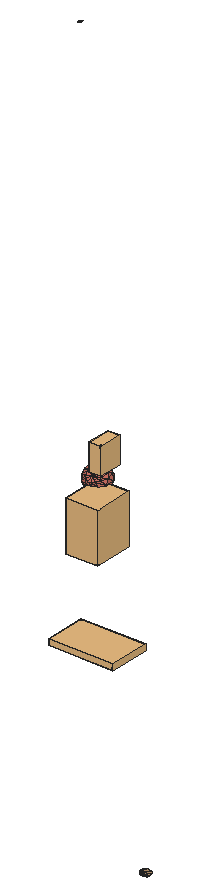
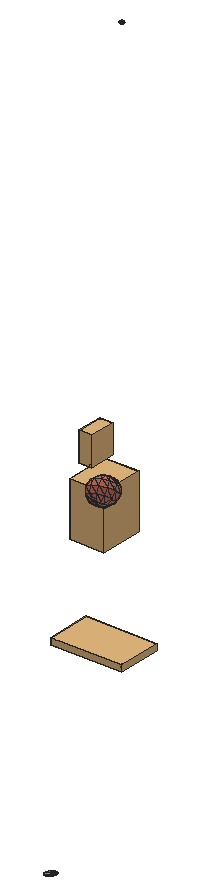
# SketchUp Ruby script. Lengths in inches.
U = 1.inch
M = Sketchup.active_model
def pt(a) = Geom::Point3d.new(a.map { |v| v * U })
def face(e, loops, mat)
  f = e.add_face(loops[0].map { |a| pt(a) })
  loops[1..].each { |l| e.add_face(l.map { |a| pt(a) }).erase! }
  f.material = f.back_material = mat if mat
  f
end
# faces: each face lists its corners as indices into pts; further lists are holes
def faces(e, pts, list, mat = nil) = list.each { |f| face(e, (f[0].is_a?(Array) ? f : [f]).map { |l| l.map { |i| pts[i] } }, mat) }
# xy, xz, yz: faces in a plane at the given z, y or x. An outline is a flat list of corners, or four numbers for a rectangle; further outlines are holes
def ring(l) = l.size == 4 ? [[l[0], l[1]], [l[2], l[1]], [l[2], l[3]], [l[0], l[3]]] : l.each_slice(2).to_a
def flat(e, list, mat, &to3) = list.each { |f| face(e, (f[0].is_a?(Array) ? f : [f]).map { |l| ring(l).map { |u, v| to3.(u, v) } }, mat) }
def xy(e, z, list, mat = nil) = flat(e, list, mat) { |x, y| [x, y, z] }
def xz(e, y, list, mat = nil) = flat(e, list, mat) { |x, z| [x, y, z] }
def yz(e, x, list, mat = nil) = flat(e, list, mat) { |y, z| [x, y, z] }
def lines(e, pts, list) = list.each { |a, b| e.add_line(pt(pts[a]), pt(pts[b])) }
# prism: a flat outline (further loops are holes) pulled along v
def prism(e, loops, v, mat = nil)
  f = face(e, loops, mat); d = Geom::Vector3d.new(v.map { |x| x * U })
  f.pushpull(f.normal.samedirection?(d) ? d.length : -d.length)
end
def box(e, o, s, mat = nil) = prism(e, [[o, [o[0] + s[0], o[1], o[2]], [o[0] + s[0], o[1] + s[1], o[2]], [o[0], o[1] + s[1], o[2]]]], [0, 0, s[2]], mat)
def at(x, y, z, deg = 0) = Geom::Transformation.translation(pt([x, y, z])) * Geom::Transformation.rotation(ORIGIN, Z_AXIS, deg.degrees)
def axes(o, x, y, z) = Geom::Transformation.new([*x, 0, *y, 0, *z, 0, *pt(o).to_a, 1])
def part(name) = M.definitions.add(name)
# library, detail: a bought-in or finely detailed component or shape, given as its bounding box
def library(name, o, s) = part(name).tap { |d| box(d.entities, o, s) }
def detail(e, o, s) = box(e.add_group.entities, o, s)
def put(e, d, t, mat = nil) = e.add_instance(d, t).tap { |i| i.material = mat if mat }
def group(e, t, mat = nil) = e.add_group.tap { |g| g.transformation = t; g.material = mat if mat }.entities
root = M.entities
M.materials.add("green").color = [174, 139, 102]
M.materials.add("vio").color = [206, 114, 100]
c1 = part("3DGeom~213_Defintion")
p = [[-61.03,-133.26,-481.34],[151.11,0,-487.05],[280.8,-170.5625,-375.28],[435.08,-14.45,-265.46],[280.8,-170.5625,-375.28],[-208.41,14.45,-465.11],
  [322.77,133.26,-362.26],[435.08,-14.45,-265.46],[-19.0625,170.56,-468.3125],[-256.82,-230.81,-346.65],[51.28,-280.97,-384.54],[280.8,-170.5625,-375.28],
  [51.28,-280.97,-384.54],[-341.91,-145.53,-337.28],[-256.82,-230.81,-346.65],[-341.91,-145.53,-337.28],[-351.36,122.58,-340.21],[-184.13,295.42,-324.09],
  [175.39,280.97,-346.03],[-424.44,-83.1,-265.17],[-341.91,-145.53,-337.28],[-424.44,-83.1,-265.17],[-191.98,-316.09,-290.76],[51.28,-280.97,-384.54],
  [98.43,-389.1,-200.66],[335.24,-295.42,-162.95],[-256.82,-230.81,-346.65],[51.28,-280.97,-384.54],[-191.98,-316.09,-290.76],[280.8,-170.5625,-375.28],
  [280.8,-170.5625,-375.28],[482.23,-122.58,-81.58],[335.24,-295.42,-162.95],[280.8,-170.5625,-375.28],[435.08,-14.45,-265.46],[322.77,133.26,-362.26],
  [472.78,145.53,-84.51],[175.39,280.97,-346.03],[407.9375,230.81,-140.4],[322.77,133.26,-362.26],[322.77,133.26,-362.26],[-256.82,-230.81,-346.65],
  [-191.98,-316.09,-290.76],[-383.8,-266.51,-119.08],[-341.91,-145.53,-337.28],[-383.8,-266.51,-119.08],[175.39,280.97,-346.03],[322.85,316.09,-131.03],
  [32.44,389.1,-221.13],[32.44,389.1,-221.13],[322.85,316.09,-131.03],[175.39,280.97,-346.03],[-482.31,-60.25,-149.64],[-351.36,122.58,-340.21],
  [-424.44,-83.1,-265.17],[-451.58,162.16,-140.11],[-351.36,122.58,-340.21],[-184.13,295.42,-324.09],[-351.36,122.58,-340.21],[-383.8,-266.51,-119.08],
  [-299.86,341.12,-93.03],[-184.13,295.42,-324.09],[-299.86,341.12,-93.03],[32.44,389.1,-221.13],[-184.13,295.42,-324.09],[-164.76,-378.52,-184.6],
  [-383.8,-266.51,-119.08],[500,83.1,21.65],[-383.8,-266.51,-119.08],[32.44,389.1,-221.13],[240.32,378.52,-58.92],[322.85,316.09,-131.03],
  [-299.86,341.12,-93.03],[-67.78,428.68,-21.03],[32.44,389.1,-221.13],[32.44,389.1,-221.13],[67.78,-428.68,21.03],[299.86,-341.12,93.03],
  [-182.45,-401.37,-56.61],[335.24,-295.42,-162.95],[451.58,-162.16,140.11],[299.86,-341.12,93.03],[335.24,-295.42,-162.95],[-500,-83.1,-21.65],
  [-383.8,-266.51,-119.08],[383.8,266.51,119.08],[-482.23,122.58,81.58],[240.32,378.52,-58.92],[-240.32,-378.52,58.92],[-240.32,-378.52,58.92],
  [-322.85,-316.09,131.03],[-383.8,-266.51,-119.08],[-407.9375,-230.81,140.4],[-383.8,-266.51,-119.08],[-472.78,-145.53,84.51],[-383.8,-266.51,-119.08],
  [-383.8,-266.51,-119.08],[-335.24,295.42,162.95],[-335.24,295.42,162.95],[-299.86,341.12,-93.03],[482.31,60.25,149.64],[182.45,401.37,56.61],
  [383.8,266.51,119.08],[-32.44,-389.1,221.14],[-240.32,-378.52,58.92],[-335.24,295.42,162.95],[-98.43,389.1,200.66],[184.13,-295.42,324.09],
  [184.13,-295.42,324.09],[164.76,378.52,184.6],[383.8,266.51,119.08],[-240.32,-378.52,58.92],[-175.39,-280.97,346.03],[-240.32,-378.52,58.92],
  [-175.39,-280.97,346.03],[-322.85,-316.09,131.03],[-435.08,14.45,265.46],[299.86,-341.12,93.03],[351.36,-122.58,340.21],[184.13,-295.42,324.09],
  [299.86,-341.12,93.03],[351.36,-122.58,340.21],[424.44,83.1,265.17],[341.91,145.53,337.28],[424.44,83.1,265.17],[256.82,230.81,346.65],
  [341.91,145.53,337.28],[191.98,316.09,290.76],[256.82,230.81,346.65],[191.98,316.09,290.76],[383.8,266.51,119.08],[-322.77,-133.26,362.26],
  [-175.39,-280.97,346.03],[424.44,83.1,265.17],[351.36,-122.58,340.21],[424.44,83.1,265.17],[-280.8,170.5625,375.28],[-280.8,170.5625,375.28],
  [-335.24,295.42,162.95],[-51.28,280.97,384.54],[-280.8,170.5625,375.28],[-32.44,-389.1,221.14],[19.0625,-170.56,468.3125],[-175.39,-280.97,346.03],
  [-32.44,-389.1,221.14],[184.13,-295.42,324.09],[351.36,-122.58,340.21],[424.44,83.1,265.17],[341.91,145.53,337.28],[-322.77,-133.26,362.26],
  [-280.8,170.5625,375.28],[-435.08,14.45,265.46],[61.03,133.26,481.34],[191.98,316.09,290.76],[-51.28,280.97,384.54],[256.82,230.81,346.65],
  [191.98,316.09,290.76],[208.41,-14.45,465.11],[-175.39,-280.97,346.03],[-151.11,0,487.05],[-322.77,-133.26,362.26],[-175.39,-280.97,346.03],
  [-322.77,-133.26,362.26],[-280.8,170.5625,375.28],[-51.28,280.97,384.54],[-280.8,170.5625,375.28],[-51.28,280.97,384.54]]
faces(c1.entities,p,[[0,1,2],[1,3,4],[5,1,0],[1,6,7],[5,8,1],[8,6,1],[9,0,10],[0,11,12],
  [13,0,14],[15,5,0],[16,8,5],[16,17,8],[8,18,6],[17,18,8],[19,5,20],[21,16,5],
  [22,23,24],[23,25,24],[26,27,28],[23,29,25],[30,31,32],[33,34,31],[35,36,34],[37,38,39],
  [40,38,36],[41,42,43],[44,41,45],[46,47,38],[17,48,18],[49,50,51],[52,53,54],[52,55,56],
  [55,57,58],[54,44,59],[55,60,61],[62,63,64],[22,24,65],[22,65,66],[34,67,31],[34,36,67],
  [52,54,68],[69,70,71],[72,73,74],[73,70,75],[65,24,76],[24,77,76],[24,25,77],[65,76,78],
  [65,78,66],[79,80,81],[82,31,80],[83,52,84],[83,55,52],[36,38,85],[38,47,85],[83,86,55],
  [86,60,55],[47,87,85],[78,88,66],[89,90,91],[90,92,93],[94,83,95],[92,94,96],[86,97,60],
  [98,73,99],[67,36,85],[31,100,80],[31,67,100],[70,101,102],[73,101,70],[78,76,103],[78,103,104],
  [94,86,83],[105,106,73],[106,101,73],[76,107,103],[76,77,108],[100,67,85],[101,109,110],[106,109,101],
  [111,103,112],[113,114,115],[94,116,86],[116,97,86],[92,116,94],[117,118,119],[120,80,121],[122,100,85],
  [123,124,85],[125,126,85],[127,128,85],[109,129,130],[90,131,92],[90,132,131],[80,133,134],[80,100,135],
  [92,131,116],[116,136,97],[137,106,138],[139,109,106],[139,129,109],[140,139,106],[141,142,143],[144,145,142],
  [146,147,148],[149,150,151],[152,153,154],[152,155,156],[145,157,142],[145,146,157],[146,148,157],[157,148,155],
  [158,159,160],[161,142,159],[157,155,152],[162,159,163],[159,164,165],[159,152,166],[142,157,152],[142,152,159]],"vio")
c2 = library("3DGeom~82_Defintion",[-311.46,-44.07,-500],[622.92,88.14,1000])
c3 = part("3DGeom~83_Defintion")
p = [[-298.62,24.62,-492.72],[-284.8,11.4,-500],[-286.34,4.79,-498.51],[-298.62,24.62,-492.72],[-286.83,18.01,-499.32],[-284.8,11.4,-500],
  [-298.62,24.62,-492.72],[-291.89,22.84,-496.66],[-286.83,18.01,-499.32],[-298.62,24.62,-492.72],[-286.34,4.79,-498.51],[-291.04,-0.05,-495.25],
  [-298.62,24.62,-492.72],[-291.04,-0.05,-495.25],[-297.64,-1.82,-491.09],[-298.62,24.62,-492.72],[-297.64,-1.82,-491.09],[-304.37,-0.05,-487.15],
  [-298.62,24.62,-492.72],[-304.37,-0.05,-487.15],[-309.43,4.79,-484.49],[-298.62,24.62,-492.72],[-309.43,4.79,-484.49],[-311.46,11.4,-483.81],
  [-298.62,24.62,-492.72],[-311.46,11.4,-483.81],[-309.92,18.01,-485.3],[-298.62,24.62,-492.72],[-309.92,18.01,-485.3],[-305.22,22.84,-488.56],
  [307.6,-38.25,479.62],[301.85,-20.79,496.17],[294.12,-44.07,483.45],[307.6,-38.25,479.62],[294.12,-44.07,483.45],[301.3,-42.51,480.25],
  [311.46,-26.61,485.98],[301.85,-20.79,496.17],[307.6,-38.25,479.62],[311.46,-26.61,485.98],[307.6,-38.25,479.62],[311.32,-32.43,481.71],
  [294.12,-44.07,483.45],[301.85,-20.79,496.17],[284.51,-38.25,493.64],[294.12,-44.07,483.45],[284.51,-38.25,493.64],[287.97,-42.51,488.35],
  [301.85,-20.79,496.17],[311.46,-26.61,485.98],[307.99,-22.35,491.27],[284.51,-38.25,493.64],[301.85,-20.79,496.17],[288.37,-26.61,500],
  [284.51,-38.25,493.64],[284.65,-32.43,497.9],[301.85,-20.79,496.17],[294.66,-22.35,499.36]]
faces(c3.entities,p,[[0,1,2],[3,4,5],[6,7,8],[9,10,11],[12,13,14],[15,16,17],[18,19,20],[21,22,23],
  [24,25,26],[27,28,29],[30,31,32],[33,34,35],[36,37,38],[39,40,41],[42,43,44],[45,46,47],
  [48,49,50],[51,52,53],[54,53,55],[56,57,53]],"green")
c4 = library("3DGeom~150_Defintion",[-440.97,-500,-219.09],[881.94,1000,438.17])
c5 = part("3DGeom~151_Defintion")
p = [[-380.69,-485.53,-210.54],[-411.26,-467,-218.1875],[-394.16,-475.51,-219.09],[-380.69,-485.53,-210.54],[-434.74,-476.74,-157.14],[-411.26,-467,-218.1875],
  [-438.29,-462.61,-191.49],[-411.26,-467,-218.1875],[-438.29,-462.61,-191.49],[-427.41,-462.28,-208.09],[-377.14,-499.67,-176.1875],[-434.74,-476.74,-157.14],
  [-380.69,-485.53,-210.54],[-377.14,-499.67,-176.1875],[-380.69,-485.53,-210.54],[-374.46,-494.375,-194.84],[-434.74,-476.74,-157.14],[-440.97,-467.9,-172.84],
  [-438.29,-462.61,-191.49],[-404.17,-495.28,-149.49],[-377.14,-499.67,-176.1875],[-388.02,-500,-159.59],[-404.17,-495.28,-149.49],[-434.74,-476.74,-157.14],
  [-404.17,-495.28,-149.49],[-421.27,-486.76,-148.6],[402.51,492.03,208.37],[431.04,458.58,149.1],[419.28,470.25,140.94],[402.51,492.03,208.37],
  [419.28,470.25,140.94],[406.85,483.28,142.92],[402.51,492.03,208.37],[406.85,483.28,142.92],[397.08,494.17,154.49],[402.51,492.03,208.37],
  [438.98,451.39,165.19],[431.04,458.58,149.1],[402.51,492.03,208.37],[397.08,494.17,154.49],[392.58,500,172.55],[402.51,492.03,208.37],
  [440.97,450.61,184.92],[438.98,451.39,165.19],[402.51,492.03,208.37],[392.58,500,172.55],[394.57,499.22,192.28],[402.51,492.03,208.37],
  [436.48,456.44,202.98],[440.97,450.61,184.92],[402.51,492.03,208.37],[426.7,467.33,214.55],[402.51,492.03,208.37],[414.27,480.36,216.53],
  [426.7,467.33,214.55]]
faces(c5.entities,p,[[0,1,2],[3,4,5],[5,4,6],[7,8,9],[10,11,12],[13,14,15],[16,17,18],[19,20,21],
  [22,11,10],[23,24,25],[26,27,28],[29,30,31],[32,33,34],[35,36,37],[38,39,40],[41,42,43],
  [44,45,46],[47,48,49],[50,51,48],[52,53,54]],"green")
c6 = part("3DGeom~137_Defintion")
p = [[-12.7,499.9,-47.63],[-12.43,498.46,-37.01],[-9.46,500,-49.08],[-9.46,500,-49.08],[-12.43,498.46,-37.01],[-5.93,499.84,-48.71],
  [-9.46,500,-49.08],[-5.93,499.84,-48.71],[-7.64,499.95,-49.12],[-12.7,499.9,-47.63],[-9.46,500,-49.08],[-11.2,499.98,-48.56],
  [-5.93,499.84,-48.71],[-12.43,498.46,-37.01],[-3.15,499.49,-46.71],[-5.93,499.84,-48.71],[-3.15,499.49,-46.71],[-4.41,499.68,-47.89],
  [-13.6875,498.66,-38.1875],[-12.43,498.46,-37.01],[-12.7,499.9,-47.63],[-13.6875,498.66,-38.1875],[-12.7,499.9,-47.63],[-13.9,499.77,-46.38],
  [-3.15,499.49,-46.71],[-12.43,498.46,-37.01],[-1.7,499.01,-43.51],[-3.15,499.49,-46.71],[-1.7,499.01,-43.51],[-2.22,499.26,-45.24],
  [-15.16,499.38,-43.18],[-13.6875,498.66,-38.1875],[-13.9,499.77,-46.38],[-15.16,499.38,-43.18],[-13.9,499.77,-46.38],[-14.73,499.59,-44.87],
  [-1.7,499.01,-43.51],[-12.43,498.46,-37.01],[-2.1,498.55,-40.03],[-1.7,499.01,-43.51],[-2.1,498.55,-40.03],[-1.67,498.77,-41.72],
  [-15.13,499.14,-41.38],[-13.6875,498.66,-38.1875],[-15.16,499.38,-43.18],[-15.13,499.14,-41.38],[-14.61,498.89,-39.66],[-13.6875,498.66,-38.1875],
  [-2.1,498.55,-40.03],[-12.43,498.46,-37.01],[-4.13,498.24,-37.26],[-2.1,498.55,-40.03],[-4.13,498.24,-37.26],[-2.9375,498.375,-38.52],
  [-4.13,498.24,-37.26],[-12.43,498.46,-37.01],[-7.375,498.15,-35.82],[-4.13,498.24,-37.26],[-7.375,498.15,-35.82],[-5.63,498.17,-36.34],
  [-7.375,498.15,-35.82],[-12.43,498.46,-37.01],[-10.9,498.31,-36.19],[-7.375,498.15,-35.82],[-10.9,498.31,-36.19],[-9.2,498.2,-35.78],
  [5.92,-499.89,57.44],[6.49,-499.97,57.1],[7.15,-500,56.9],[5.92,-499.89,57.44],[7.15,-500,56.9],[6.04,-498.77,61.29],
  [7.15,-500,56.9],[8.48,-499.91,57.02],[6.04,-498.77,61.29],[7.15,-500,56.9],[7.84,-499.98,56.88],[8.48,-499.91,57.02],
  [8.48,-499.91,57.02],[9.54,-499.66,57.73],[6.04,-498.77,61.29],[8.48,-499.91,57.02],[9.06,-499.8,57.31],[9.54,-499.66,57.73],
  [5.5625,-498.91,60.87],[5.47,-499.78,57.9],[5.92,-499.89,57.44],[5.5625,-498.91,60.87],[5.92,-499.89,57.44],[6.04,-498.77,61.29],
  [9.54,-499.66,57.73],[10.09,-499.31,58.88],[6.04,-498.77,61.29],[9.54,-499.66,57.73],[9.89,-499.5,58.26],[10.09,-499.31,58.88],
  [5,-499.46,59.0625],[5.16,-499.63,58.45],[5.47,-499.78,57.9],[5,-499.46,59.0625],[5.47,-499.78,57.9],[5.5625,-498.91,60.87],
  [10.09,-499.31,58.88],[9.94,-498.95,60.15],[6.04,-498.77,61.29],[10.09,-499.31,58.88],[10.1,-499.12,59.53],[9.94,-498.95,60.15],
  [5.5625,-498.91,60.87],[5.01,-499.27,59.72],[5,-499.46,59.0625],[5.5625,-498.91,60.87],[5.21,-499.08,60.34],[5.01,-499.27,59.72],
  [9.94,-498.95,60.15],[9.17,-498.68,61.16],[6.04,-498.77,61.29],[9.94,-498.95,60.15],[9.625,-498.8,60.7],[9.17,-498.68,61.16],
  [9.17,-498.68,61.16],[7.95,-498.58,61.7],[6.04,-498.77,61.29],[9.17,-498.68,61.16],[8.61,-498.61,61.5],[7.95,-498.58,61.7],
  [7.95,-498.58,61.7],[6.62,-498.66,61.58],[6.04,-498.77,61.29],[7.95,-498.58,61.7],[7.26,-498.6,61.72],[6.62,-498.66,61.58]]
faces(c6.entities,p,[[0,1,2],[3,4,5],[6,7,8],[9,10,11],[12,13,14],[15,16,17],[18,19,20],[21,22,23],
  [24,25,26],[27,28,29],[30,31,32],[33,34,35],[36,37,38],[39,40,41],[42,43,44],[45,46,47],
  [48,49,50],[51,52,53],[54,55,56],[57,58,59],[60,61,62],[63,64,65],[66,67,68],[69,70,71],
  [72,73,74],[75,76,77],[78,79,80],[81,82,83],[84,85,86],[87,88,89],[90,91,92],[93,94,95],
  [96,97,98],[99,100,101],[102,103,104],[105,106,107],[108,109,110],[111,112,113],[114,115,116],[117,118,119],
  [120,121,122],[123,124,125],[126,127,128],[129,130,131]],"green")
c7 = library("3DGeom~84_Defintion",[-394.11,-500,-321.29],[788.22,1000,642.58])
c8 = part("3DGeom~85_Defintion")
p = [[-385.68,493.0625,-287],[-375.2,479.16,-321.29],[-384.38,476.9375,-316.78],[-385.68,493.0625,-287],[-366.22,483.875,-321.2],[-375.2,479.16,-321.29],
  [-385.68,493.0625,-287],[-359.85,489.82,-316.53],[-366.22,483.875,-321.2],[-385.68,493.0625,-287],[-384.38,476.9375,-316.78],[-391.31,477.81,-308.86],
  [-385.68,493.0625,-287],[-357.79,495.41,-308.52],[-359.85,489.82,-316.53],[-385.68,493.0625,-287],[-391.31,477.81,-308.86],[-394.11,481.53,-299.68],
  [-385.68,493.0625,-287],[-360.59,499.13,-299.34],[-357.79,495.41,-308.52],[-385.68,493.0625,-287],[-394.11,481.53,-299.68],[-392.05,487.11,-291.68],
  [-385.68,493.0625,-287],[-367.52,500,-291.43],[-360.59,499.13,-299.34],[-385.68,493.0625,-287],[-376.7,497.78,-286.91],[-367.52,500,-291.43],
  [382.1,-486.4,280.5],[375.41,-492.22,320.16],[367.13,-497.09,286.29],[382.1,-486.4,280.5],[367.13,-497.09,286.29],[373.98,-492.12,280.77],
  [393.73,-478.62,294.54],[393.73,-478.62,294.54],[382.1,-486.4,280.5],[389.33,-481.46,285.53],[367.13,-497.09,286.29],[363.79,-500,306.12],
  [363.4,-499.97,295.5625],[367.13,-497.09,286.29],[375.41,-492.22,320.16],[363.79,-500,306.12],[390.38,-481.53,314.37],[390.38,-481.53,314.37],
  [393.73,-478.62,294.54],[394.11,-478.65,305.09],[375.41,-492.22,320.16],[368.18,-497.16,315.12],[363.79,-500,306.12],[375.41,-492.22,320.16],
  [390.38,-481.53,314.37],[383.54,-486.5,319.88]]
faces(c8.entities,p,[[0,1,2],[3,4,5],[6,7,8],[9,10,11],[12,13,14],[15,16,17],[18,19,20],[21,22,23],
  [24,25,26],[27,28,29],[30,31,32],[33,34,35],[36,31,30],[37,38,39],[40,41,42],[43,44,45],
  [46,31,36],[47,48,49],[50,51,52],[53,54,55]],"green")
g1 = group(root,at(15.3125,38.42,26.21))
put(g1,c1,axes([-1.84,0.51,8.4],[0,0.00038,0],[0,0,-0.00038],[-0.00038,0,0]),"vio")
g2 = group(root,at(15.3125,38.42,26.21))
put(g2,c2,axes([-1.65,0.26,6.38],[0,0.00095,0],[0,0,-0.00095],[-0.00095,0,0]),"green")
put(g2,c3,axes([-1.65,0.26,6.38],[0,0.00095,0],[0,0,-0.00095],[-0.00095,0,0]),"green")
g3 = group(root,at(15.3125,38.42,26.21))
put(g3,c4,axes([-1.63,0.37,8.85],[0,0.00039,0],[0,0,-0.00039],[-0.00039,0,0]),"green")
put(g3,c5,axes([-1.63,0.37,8.85],[0,0.00039,0],[0,0,-0.00039],[-0.00039,0,0]),"green")
put(root,c6,axes([13.77,38.96,35.07],[0,0.01074,0],[0,0,-0.01074],[-0.01074,0,0]),"green")
g4 = group(root,at(15.3125,38.42,26.21))
put(g4,c7,axes([-1.61,0.21,8.02],[0,0.00073,0],[0,0,-0.00073],[-0.00073,0,0]),"green")
put(g4,c8,axes([-1.61,0.21,8.02],[0,0.00073,0],[0,0,-0.00073],[-0.00073,0,0]),"green")
